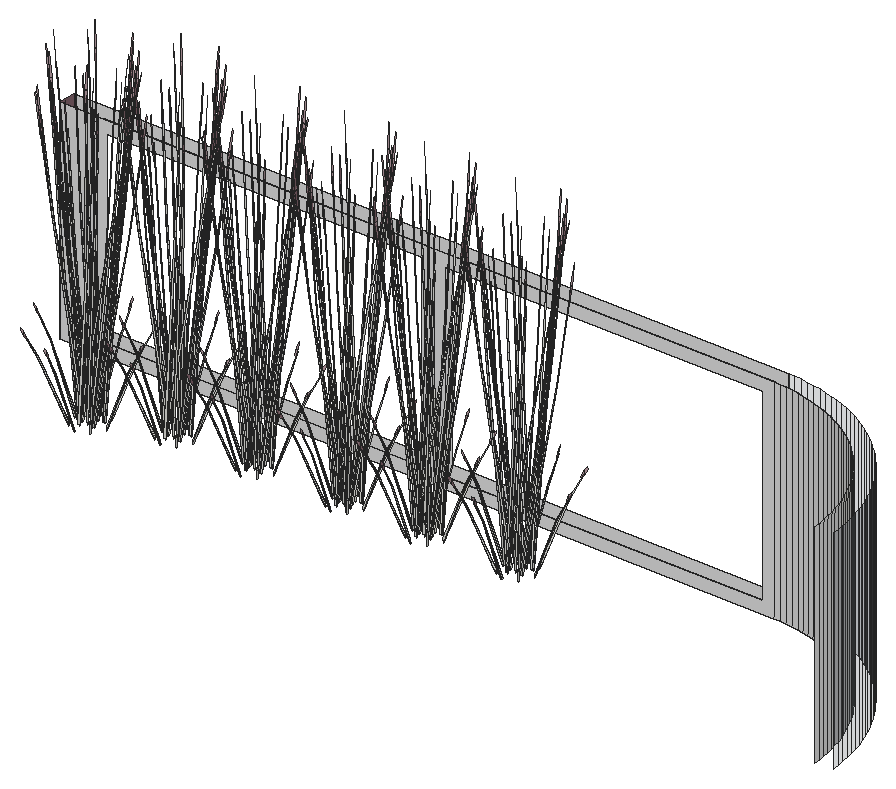
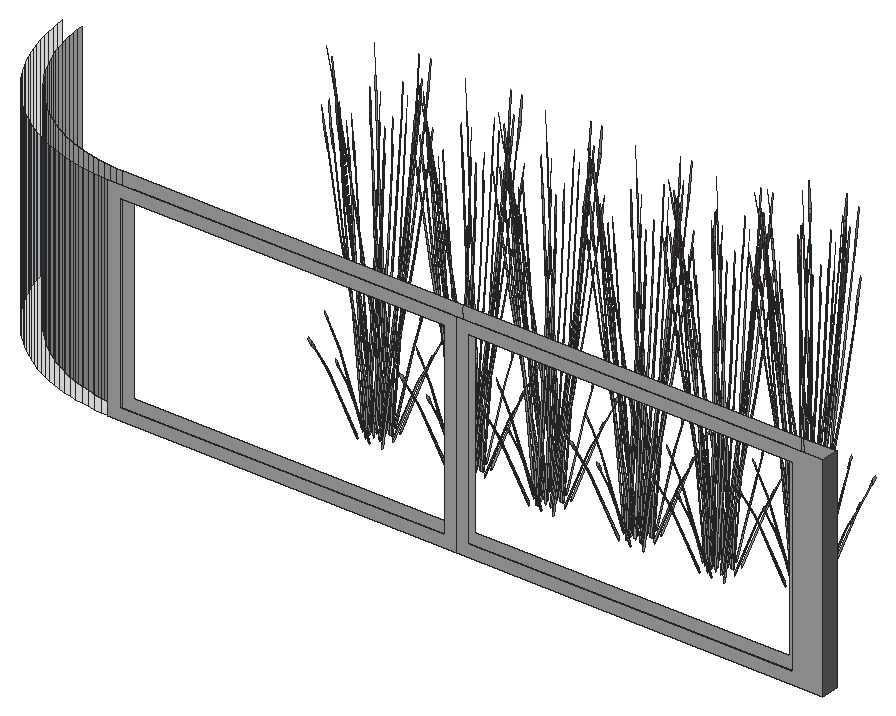
# SketchUp Ruby script. Lengths in inches.
U = 1.inch
M = Sketchup.active_model
def pt(a) = Geom::Point3d.new(a.map { |v| v * U })
def face(e, loops, mat)
  f = e.add_face(loops[0].map { |a| pt(a) })
  loops[1..].each { |l| e.add_face(l.map { |a| pt(a) }).erase! }
  f.material = f.back_material = mat if mat
  f
end
# faces: each face lists its corners as indices into pts; further lists are holes
def faces(e, pts, list, mat = nil) = list.each { |f| face(e, (f[0].is_a?(Array) ? f : [f]).map { |l| l.map { |i| pts[i] } }, mat) }
# xy, xz, yz: faces in a plane at the given z, y or x. An outline is a flat list of corners, or four numbers for a rectangle; further outlines are holes
def ring(l) = l.size == 4 ? [[l[0], l[1]], [l[2], l[1]], [l[2], l[3]], [l[0], l[3]]] : l.each_slice(2).to_a
def flat(e, list, mat, &to3) = list.each { |f| face(e, (f[0].is_a?(Array) ? f : [f]).map { |l| ring(l).map { |u, v| to3.(u, v) } }, mat) }
def xy(e, z, list, mat = nil) = flat(e, list, mat) { |x, y| [x, y, z] }
def xz(e, y, list, mat = nil) = flat(e, list, mat) { |x, z| [x, y, z] }
def yz(e, x, list, mat = nil) = flat(e, list, mat) { |y, z| [x, y, z] }
def lines(e, pts, list) = list.each { |a, b| e.add_line(pt(pts[a]), pt(pts[b])) }
# prism: a flat outline (further loops are holes) pulled along v
def prism(e, loops, v, mat = nil)
  f = face(e, loops, mat); d = Geom::Vector3d.new(v.map { |x| x * U })
  f.pushpull(f.normal.samedirection?(d) ? d.length : -d.length)
end
def box(e, o, s, mat = nil) = prism(e, [[o, [o[0] + s[0], o[1], o[2]], [o[0] + s[0], o[1] + s[1], o[2]], [o[0], o[1] + s[1], o[2]]]], [0, 0, s[2]], mat)
def at(x, y, z, deg = 0) = Geom::Transformation.translation(pt([x, y, z])) * Geom::Transformation.rotation(ORIGIN, Z_AXIS, deg.degrees)
def axes(o, x, y, z) = Geom::Transformation.new([*x, 0, *y, 0, *z, 0, *pt(o).to_a, 1])
def part(name) = M.definitions.add(name)
# library, detail: a bought-in or finely detailed component or shape, given as its bounding box
def library(name, o, s) = part(name).tap { |d| box(d.entities, o, s) }
def detail(e, o, s) = box(e.add_group.entities, o, s)
def put(e, d, t, mat = nil) = e.add_instance(d, t).tap { |i| i.material = mat if mat }
def group(e, t, mat = nil) = e.add_group.tap { |g| g.transformation = t; g.material = mat if mat }.entities
root = M.entities
M.materials.add("Glass_Basic_01").color = [105, 113, 122]
M.materials["Glass_Basic_01"].alpha = 0.25
M.materials.add("LightPink_Translucent").color = [144, 107, 117]
M.materials["LightPink_Translucent"].alpha = 0.75
M.materials.add("M01_Silver_Fog").color = [224, 224, 224]
M.materials.add("M06_Steel_Smoke").color = [114, 114, 114]
c1 = part("blade")
p = [[2.15,0.21,22],[0,0.17,0],[0.09,0.45,0],[2.18,0.31,22],[2.29,0.31,22],[0.38,0.45,0],
  [2.48,0.24,33],[2.49,0.24,33],[2.48,0.22,33]]
faces(c1.entities,p,[[0,1,2,3],[4,5,2,3],[6,3,4,7],[8,0,3,6]])
c2 = part("seeds")
p = [[0.3,-0.1,1.38],[-0.01,-0.03,1.59],[-0.01,-0.03,0.03],[0.14,-0.07,-0.07],[0.29,-0.03,3],[0.15,0.01,3.11]]
faces(c2.entities,p,[[0,1,2,3],[1,0,4,5]],"LightPink_Translucent")
c3 = part("blade with seeds")
put(c3.entities,c1,at(0,0,0))
put(c3.entities,c2,axes([2.4,0.25,30.99],[1.5799,-0.05474,1.17369],[-0.12525,1.92788,0.29478],[-0.07173,-0.02425,1.56792]))
xz(root,465.98,[[355.17,396,355.18,432]],"Glass_Basic_01")
xz(root,474,[[210,396,215.53,432],[215.53,396,216,432],[[216,396,273.49,432],[218,398,271.49,430]],[[273.49,396,331.45,432],[275.49,398,329.45,430]]],"M01_Silver_Fog")
xz(root,477,[[[210,396,272.25,432],[215,398,270.25,430]],[[272.25,396,331.5,432],[274.25,398,329.5,430]]],"M01_Silver_Fog")
yz(root,210,[[474,396,477,432]],"M06_Steel_Smoke")
yz(root,358.13,[[462.03,396,462.04,432]],"Glass_Basic_01")
p = [[360.01,447.89,396],[360.11,446.78,396],[360.11,446.78,432],[360.01,447.89,432],[363.1,447,396],[362.99,448.22,396],
  [362.99,448.22,432],[363.1,447,432],[359.87,449,396],[359.87,449,432],[362.83,449.44,396],[362.83,449.44,432],
  [359.68,450.1,396],[359.68,450.1,432],[362.63,450.66,396],[362.63,450.66,432],[359.45,451.2,396],[359.45,451.2,432],
  [362.38,451.86,396],[362.38,451.86,432],[359.18,452.28,396],[359.18,452.28,432],[362.08,453.06,396],[362.08,453.06,432],
  [358.875,453.35,396],[358.875,453.35,432],[361.74,454.24,396],[361.74,454.24,432],[358.52,454.41,396],[358.52,454.41,432],
  [361.35,455.41,396],[361.35,455.41,432],[358.13,455.46,396],[358.13,455.46,432],[360.92,456.5625,396],[360.92,456.5625,432],
  [357.7,456.49,396],[357.7,456.49,432],[357.23,457.5,396],[357.23,457.5,432],[360.45,457.7,396],[360.45,457.7,432],
  [356.73,458.5,396],[356.73,458.5,432],[359.93,458.82,396],[359.93,458.82,432],[356.18,459.47,396],[356.18,459.47,432],
  [359.37,459.91,396],[359.37,459.91,432],[355.6,460.43,396],[355.6,460.43,432],[358.77,460.99,396],[358.77,460.99,432],
  [354.98,461.36,396],[354.98,461.36,432],[358.13,462.03,396],[358.13,462.03,432],[354.33,462.26,396],[354.33,462.26,432],
  [358.13,462.04,396],[357.45,463.0625,396],[357.45,463.0625,432],[358.13,462.04,432],[353.64,463.14,396],[353.64,463.14,432],
  [352.92,464,396],[352.92,464,432],[356.73,464.0625,396],[356.73,464.0625,432],[352.17,464.83,396],[352.17,464.83,432],
  [355.97,465.03,396],[355.97,465.03,432],[351.39,465.62,396],[351.39,465.62,432],[355.18,465.98,396],[355.18,465.98,432],
  [350.58,466.39,396],[350.58,466.39,432],[355.17,465.98,396],[354.35,466.89,396],[354.35,466.89,432],[355.17,465.98,432],
  [349.74,467.125,396],[349.74,467.125,432],[353.49,467.76,396],[353.49,467.76,432],[348.87,467.83,396],[348.87,467.83,432],
  [347.97,468.5,396],[347.97,468.5,432],[352.59,468.61,396],[352.59,468.61,432],[347.05,469.13,396],[347.05,469.13,432],
  [351.67,469.42,396],[351.67,469.42,432],[346.11,469.73,396],[346.11,469.73,432],[350.71,470.19,396],[350.71,470.19,432],
  [345.15,470.29,396],[345.15,470.29,432],[349.72,470.93,396],[349.72,470.93,432],[344.16,470.82,396],[344.16,470.82,432],
  [343.16,471.3,396],[343.16,471.3,432],[348.71,471.63,396],[348.71,471.63,432],[342.13,471.75,396],[342.13,471.75,432],
  [347.67,472.29,396],[347.67,472.29,432],[341.09,472.16,396],[341.09,472.16,432],[340.04,472.53,396],[340.04,472.53,432],
  [346.61,472.91,396],[346.61,472.91,432],[338.97,472.86,396],[338.97,472.86,432],[337.89,473.15,396],[337.89,473.15,432],
  [345.52,473.49,396],[345.52,473.49,432],[336.8,473.4,396],[336.8,473.4,432],[335.71,473.6,396],[335.71,473.6,432],
  [344.41,474.03,396],[344.41,474.03,432],[334.6,473.77,396],[334.6,473.77,432],[333.49,473.89,396],[333.49,473.89,432],
  [332.38,473.97,396],[332.38,473.97,432],[331.45,474,396],[331.45,474,432],[343.29,474.52,396],[343.29,474.52,432],
  [342.14,474.97,396],[342.14,474.97,432],[340.98,475.38,396],[340.98,475.38,432],[339.8,475.75,396],[339.8,475.75,432],
  [338.61,476.0625,396],[338.61,476.0625,432],[337.41,476.34,396],[337.41,476.34,432],[336.2,476.5625,396],[336.2,476.5625,432],
  [334.99,476.74,396],[334.99,476.74,432],[333.76,476.88,396],[333.76,476.88,432],[332.53,476.97,396],[332.53,476.97,432],
  [331.5,477,396],[331.5,477,432]]
faces(root,p,[[0,1,2,3],[8,0,3,9],[12,8,9,13],[16,12,13,17],[20,16,17,21],[24,20,21,25],[28,24,25,29],[32,28,29,33],
  [36,32,33,37],[38,36,37,39],[42,38,39,43],[46,42,43,47],[50,46,47,51],[54,50,51,55],[58,54,55,59],[64,58,59,65],
  [66,64,65,67],[70,66,67,71],[74,70,71,75],[78,74,75,79],[84,78,79,85],[88,84,85,89],[90,88,89,91],[94,90,91,95],
  [98,94,95,99],[102,98,99,103],[106,102,103,107],[108,106,107,109],[112,108,109,113],[116,112,113,117],[118,116,117,119],[122,118,119,123],
  [124,122,123,125],[128,124,125,129],[130,128,129,131],[134,130,131,135],[136,134,135,137],[138,136,137,139],[140,138,139,141]],"M01_Silver_Fog")
faces(root,p,[[4,5,6,7],[5,10,11,6],[10,14,15,11],[14,18,19,15],[18,22,23,19],[22,26,27,23],[26,30,31,27],[30,34,35,31],
  [34,40,41,35],[40,44,45,41],[44,48,49,45],[48,52,53,49],[52,56,57,53],[60,61,62,63],[61,68,69,62],[68,72,73,69],
  [72,76,77,73],[80,81,82,83],[81,86,87,82],[86,92,93,87],[92,96,97,93],[96,100,101,97],[100,104,105,101],[104,110,111,105],
  [110,114,115,111],[114,120,121,115],[120,126,127,121],[126,132,133,127],[132,142,143,133],[142,144,145,143],[144,146,147,145],[146,148,149,147],
  [148,150,151,149],[150,152,153,151],[152,154,155,153],[154,156,157,155],[156,158,159,157],[158,160,161,159],[160,162,163,161]],"Glass_Basic_01")
put(root,c3,axes([228.93,453.59,397.49],[-0.08428,0.0194,1.76342],[-0.46606,-0.21841,-0.26939],[0.00782,-0.18218,0.30037]))
put(root,c3,axes([227.42,454.26,397.49],[-0.04867,0.07094,1.76342],[-0.49185,0.15296,-0.26939],[-0.11882,-0.13915,0.30037]))
put(root,c3,axes([228.23,456.2,398.1],[-0.20635,-0.55225,-0.69835],[0.59439,-0.19889,-0.18329],[-0.02281,-0.18701,1.54149]))
put(root,c3,axes([230.99,454.52,397.49],[-0.0752,-0.04243,1.76342],[-0.19317,-0.47398,-0.26939],[0.13031,-0.12863,0.30037]))
put(root,c3,axes([227.01,456.13,398.02],[0,-0.53854,-0.49651],[0.56215,0,0],[0,-0.12266,1.57504]))
put(root,c3,axes([228.58,454.53,398.02],[0.47024,-0.26927,-0.49651],[0.28107,0.48284,0],[0.1071,-0.06133,1.57504]))
put(root,c3,axes([229.13,455.64,398.06],[0.33843,-0.40479,-0.62353],[0.42041,0.36705,-0.16365],[0.13561,-0.10098,1.37633]))
put(root,c3,axes([228.54,456.35,398.21],[0.24378,-0.48527,-0.44739],[0.50654,0.23354,0.21531],[0,-0.11186,1.43643]))
put(root,c3,axes([228.77,456.11,398.67],[-0.05855,-0.61451,-0.29095],[0.60981,-0.03716,-0.50002],[0.10738,-0.08185,1.59708]))
put(root,c3,axes([227.26,456.14,398.03],[0.35073,-0.33601,-0.30978],[0.35073,0.33601,0.30978],[0,-0.10823,1.38974]))
put(root,c3,axes([228.48,456.75,398.67],[-0.56585,-0.25696,-0.29095],[0.27246,-0.54236,-0.50002],[-0.01778,-0.13316,1.59708]))
put(root,c3,axes([228.6875,454.75,398.03],[0.46876,0.13325,-0.30978],[-0.11803,0.46926,0.30978],[0.0945,-0.05411,1.38974]))
put(root,c3,axes([240.17,457.83,397.49],[-0.08428,0.0194,1.76342],[-0.46606,-0.21841,-0.26939],[0.00782,-0.18218,0.30037]))
put(root,c3,axes([253.88,457.83,397.49],[-0.08428,0.0194,1.76342],[-0.46606,-0.21841,-0.26939],[0.00782,-0.18218,0.30037]))
put(root,c3,axes([269.125,457.83,397.49],[-0.08428,0.0194,1.76342],[-0.46606,-0.21841,-0.26939],[0.00782,-0.18218,0.30037]))
put(root,c3,axes([282.74,457.83,397.49],[-0.08428,0.0194,1.76342],[-0.46606,-0.21841,-0.26939],[0.00782,-0.18218,0.30037]))
put(root,c3,axes([298.27,457.83,397.49],[-0.08428,0.0194,1.76342],[-0.46606,-0.21841,-0.26939],[0.00782,-0.18218,0.30037]))
put(root,c3,axes([228.58,457.0625,398.21],[-0.30184,-0.45202,-0.44739],[0.45719,-0.31831,0.21531],[-0.09768,-0.05593,1.43643]))
put(root,c3,axes([228.3125,457.24,398.06],[-0.52267,-0.08829,-0.62353],[0.11029,-0.54463,-0.16365],[-0.15598,-0.06599,1.37633]))
put(root,c3,axes([228.19,455.71,397.59],[-0.49456,0.21561,1.28929],[-0.15741,-0.61865,0.50096],[0.30369,0.01029,1.46642]))
put(root,c3,axes([238.66,458.5,397.49],[-0.04867,0.07094,1.76342],[-0.49185,0.15296,-0.26939],[-0.11882,-0.13915,0.30037]))
put(root,c3,axes([252.37,458.5,397.49],[-0.04867,0.07094,1.76342],[-0.49185,0.15296,-0.26939],[-0.11882,-0.13915,0.30037]))
put(root,c3,axes([267.62,458.5,397.49],[-0.04867,0.07094,1.76342],[-0.49185,0.15296,-0.26939],[-0.11882,-0.13915,0.30037]))
put(root,c3,axes([281.23,458.5,397.49],[-0.04867,0.07094,1.76342],[-0.49185,0.15296,-0.26939],[-0.11882,-0.13915,0.30037]))
put(root,c3,axes([296.76,458.5,397.49],[-0.04867,0.07094,1.76342],[-0.49185,0.15296,-0.26939],[-0.11882,-0.13915,0.30037]))
put(root,c3,axes([232.05,456.55,397.49],[-0.02626,-0.08176,1.76342],[0.18213,-0.47826,-0.26939],[0.18372,-0.00688,0.30037]))
put(root,c3,axes([239.48,460.45,398.1],[-0.20635,-0.55225,-0.69835],[0.59439,-0.19889,-0.18329],[-0.02281,-0.18701,1.54149]))
put(root,c3,axes([253.18,460.45,398.1],[-0.20635,-0.55225,-0.69835],[0.59439,-0.19889,-0.18329],[-0.02281,-0.18701,1.54149]))
put(root,c3,axes([268.43,460.45,398.1],[-0.20635,-0.55225,-0.69835],[0.59439,-0.19889,-0.18329],[-0.02281,-0.18701,1.54149]))
put(root,c3,axes([282.04,460.45,398.1],[-0.20635,-0.55225,-0.69835],[0.59439,-0.19889,-0.18329],[-0.02281,-0.18701,1.54149]))
put(root,c3,axes([297.58,460.45,398.1],[-0.20635,-0.55225,-0.69835],[0.59439,-0.19889,-0.18329],[-0.02281,-0.18701,1.54149]))
put(root,c3,axes([242.23,458.76,397.49],[-0.0752,-0.04243,1.76342],[-0.19317,-0.47398,-0.26939],[0.13031,-0.12863,0.30037]))
put(root,c3,axes([255.94,458.76,397.49],[-0.0752,-0.04243,1.76342],[-0.19317,-0.47398,-0.26939],[0.13031,-0.12863,0.30037]))
put(root,c3,axes([271.19,458.76,397.49],[-0.0752,-0.04243,1.76342],[-0.19317,-0.47398,-0.26939],[0.13031,-0.12863,0.30037]))
put(root,c3,axes([284.8,458.76,397.49],[-0.0752,-0.04243,1.76342],[-0.19317,-0.47398,-0.26939],[0.13031,-0.12863,0.30037]))
put(root,c3,axes([300.33,458.76,397.49],[-0.0752,-0.04243,1.76342],[-0.19317,-0.47398,-0.26939],[0.13031,-0.12863,0.30037]))
put(root,c3,axes([226.63,456.47,397.49],[0.01274,0.08487,1.76342],[-0.25688,0.44323,-0.26939],[-0.18246,-0.02234,0.30037]))
put(root,c3,axes([227.76,458.07,398.03],[-0.11803,-0.46926,-0.30978],[0.46876,-0.13325,0.30978],[-0.0945,-0.05411,1.38974]))
put(root,c3,axes([229.47,456.03,398.67],[0.5073,-0.35754,-0.29095],[0.33735,0.5052,-0.50002],[0.12516,0.05131,1.59708]))
put(root,c3,axes([227.625,458.27,398.02],[-0.47024,-0.26927,-0.49651],[0.28107,-0.48284,0],[-0.1071,-0.06133,1.57504]))
put(root,c3,axes([230.75,455.08,398.02],[0.47024,0.26927,-0.49651],[-0.28107,0.48284,0],[0.1071,0.06133,1.57504]))
put(root,c3,axes([228.9,457.32,398.67],[-0.5073,0.35754,-0.29095],[-0.33735,-0.5052,-0.50002],[-0.12516,-0.05131,1.59708]))
put(root,c3,axes([230.62,455.28,398.03],[0.11803,0.46926,-0.30978],[-0.46876,0.13325,0.30978],[0.0945,0.05411,1.38974]))
put(root,c3,axes([238.26,460.375,398.02],[0,-0.53854,-0.49651],[0.56215,0,0],[0,-0.12266,1.57504]))
put(root,c3,axes([251.97,460.375,398.02],[0,-0.53854,-0.49651],[0.56215,0,0],[0,-0.12266,1.57504]))
put(root,c3,axes([267.22,460.375,398.02],[0,-0.53854,-0.49651],[0.56215,0,0],[0,-0.12266,1.57504]))
put(root,c3,axes([280.83,460.375,398.02],[0,-0.53854,-0.49651],[0.56215,0,0],[0,-0.12266,1.57504]))
put(root,c3,axes([296.36,460.375,398.02],[0,-0.53854,-0.49651],[0.56215,0,0],[0,-0.12266,1.57504]))
put(root,c3,axes([239.82,458.78,398.02],[0.47024,-0.26927,-0.49651],[0.28107,0.48284,0],[0.1071,-0.06133,1.57504]))
put(root,c3,axes([253.53,458.78,398.02],[0.47024,-0.26927,-0.49651],[0.28107,0.48284,0],[0.1071,-0.06133,1.57504]))
put(root,c3,axes([268.78,458.78,398.02],[0.47024,-0.26927,-0.49651],[0.28107,0.48284,0],[0.1071,-0.06133,1.57504]))
put(root,c3,axes([282.39,458.78,398.02],[0.47024,-0.26927,-0.49651],[0.28107,0.48284,0],[0.1071,-0.06133,1.57504]))
put(root,c3,axes([297.92,458.78,398.02],[0.47024,-0.26927,-0.49651],[0.28107,0.48284,0],[0.1071,-0.06133,1.57504]))
put(root,c3,axes([230.0625,456.11,398.06],[0.52267,0.08829,-0.62353],[-0.11029,0.54463,-0.16365],[0.15598,0.06599,1.37633]))
put(root,c3,axes([240.38,459.88,398.06],[0.33843,-0.40479,-0.62353],[0.42041,0.36705,-0.16365],[0.13561,-0.10098,1.37633]))
put(root,c3,axes([254.09,459.88,398.06],[0.33843,-0.40479,-0.62353],[0.42041,0.36705,-0.16365],[0.13561,-0.10098,1.37633]))
put(root,c3,axes([269.33,459.88,398.06],[0.33843,-0.40479,-0.62353],[0.42041,0.36705,-0.16365],[0.13561,-0.10098,1.37633]))
put(root,c3,axes([282.95,459.88,398.06],[0.33843,-0.40479,-0.62353],[0.42041,0.36705,-0.16365],[0.13561,-0.10098,1.37633]))
put(root,c3,axes([298.48,459.88,398.06],[0.33843,-0.40479,-0.62353],[0.42041,0.36705,-0.16365],[0.13561,-0.10098,1.37633]))
put(root,c3,axes([239.79,460.59,398.21],[0.24378,-0.48527,-0.44739],[0.50654,0.23354,0.21531],[0,-0.11186,1.43643]))
put(root,c3,axes([253.5,460.59,398.21],[0.24378,-0.48527,-0.44739],[0.50654,0.23354,0.21531],[0,-0.11186,1.43643]))
put(root,c3,axes([268.75,460.59,398.21],[0.24378,-0.48527,-0.44739],[0.50654,0.23354,0.21531],[0,-0.11186,1.43643]))
put(root,c3,axes([282.36,460.59,398.21],[0.24378,-0.48527,-0.44739],[0.50654,0.23354,0.21531],[0,-0.11186,1.43643]))
put(root,c3,axes([297.89,460.59,398.21],[0.24378,-0.48527,-0.44739],[0.50654,0.23354,0.21531],[0,-0.11186,1.43643]))
put(root,c3,axes([238.5,460.39,398.03],[0.35073,-0.33601,-0.30978],[0.35073,0.33601,0.30978],[0,-0.10823,1.38974]))
put(root,c3,axes([252.21,460.39,398.03],[0.35073,-0.33601,-0.30978],[0.35073,0.33601,0.30978],[0,-0.10823,1.38974]))
put(root,c3,axes([267.46,460.39,398.03],[0.35073,-0.33601,-0.30978],[0.35073,0.33601,0.30978],[0,-0.10823,1.38974]))
put(root,c3,axes([281.07,460.39,398.03],[0.35073,-0.33601,-0.30978],[0.35073,0.33601,0.30978],[0,-0.10823,1.38974]))
put(root,c3,axes([296.6,460.39,398.03],[0.35073,-0.33601,-0.30978],[0.35073,0.33601,0.30978],[0,-0.10823,1.38974]))
put(root,c3,axes([229.79,456.28,398.21],[0.30184,0.45202,-0.44739],[-0.45719,0.31831,0.21531],[0.09768,0.05593,1.43643]))
put(root,c3,axes([239.93,458.99,398.03],[0.46876,0.13325,-0.30978],[-0.11803,0.46926,0.30978],[0.0945,-0.05411,1.38974]))
put(root,c3,axes([253.64,458.99,398.03],[0.46876,0.13325,-0.30978],[-0.11803,0.46926,0.30978],[0.0945,-0.05411,1.38974]))
put(root,c3,axes([268.89,458.99,398.03],[0.46876,0.13325,-0.30978],[-0.11803,0.46926,0.30978],[0.0945,-0.05411,1.38974]))
put(root,c3,axes([282.5,458.99,398.03],[0.46876,0.13325,-0.30978],[-0.11803,0.46926,0.30978],[0.0945,-0.05411,1.38974]))
put(root,c3,axes([298.03,458.99,398.03],[0.46876,0.13325,-0.30978],[-0.11803,0.46926,0.30978],[0.0945,-0.05411,1.38974]))
put(root,c3,axes([229.23,457.39,398.21],[-0.54562,0.03324,-0.44739],[-0.04934,-0.55185,0.21531],[-0.09768,0.05593,1.43643]))
put(root,c3,axes([229.6875,458.6,398.03],[-0.46876,-0.13325,-0.30978],[0.11803,-0.46926,0.30978],[-0.0945,0.05411,1.38974]))
put(root,c3,axes([229.89,456.59,398.67],[0.56585,0.25696,-0.29095],[-0.27246,0.54236,-0.50002],[0.01778,0.13316,1.59708]))
put(root,c3,axes([239.83,461.31,398.21],[-0.30184,-0.45202,-0.44739],[0.45719,-0.31831,0.21531],[-0.09768,-0.05593,1.43643]))
put(root,c3,axes([253.53,461.31,398.21],[-0.30184,-0.45202,-0.44739],[0.45719,-0.31831,0.21531],[-0.09768,-0.05593,1.43643]))
put(root,c3,axes([268.78,461.31,398.21],[-0.30184,-0.45202,-0.44739],[0.45719,-0.31831,0.21531],[-0.09768,-0.05593,1.43643]))
put(root,c3,axes([282.4,461.31,398.21],[-0.30184,-0.45202,-0.44739],[0.45719,-0.31831,0.21531],[-0.09768,-0.05593,1.43643]))
put(root,c3,axes([297.93,461.31,398.21],[-0.30184,-0.45202,-0.44739],[0.45719,-0.31831,0.21531],[-0.09768,-0.05593,1.43643]))
put(root,c3,axes([231.12,457.2,398.03],[-0.35073,0.33601,-0.30978],[-0.35073,-0.33601,0.30978],[0,0.10823,1.38974]))
put(root,c3,axes([229.61,457.24,398.67],[0.05855,0.61451,-0.29095],[-0.60981,0.03716,-0.50002],[-0.10738,0.08185,1.59708]))
put(root,c3,axes([229.83,457,398.21],[-0.24378,0.48527,-0.44739],[-0.50654,-0.23354,0.21531],[0,0.11186,1.43643]))
put(root,c3,axes([229.24,457.71,398.06],[-0.33843,0.40479,-0.62353],[-0.42041,-0.36705,-0.16365],[-0.13561,0.10098,1.37633]))
put(root,c3,axes([239.56,461.48,398.06],[-0.52267,-0.08829,-0.62353],[0.11029,-0.54463,-0.16365],[-0.15598,-0.06599,1.37633]))
put(root,c3,axes([253.26,461.48,398.06],[-0.52267,-0.08829,-0.62353],[0.11029,-0.54463,-0.16365],[-0.15598,-0.06599,1.37633]))
put(root,c3,axes([268.51,461.48,398.06],[-0.52267,-0.08829,-0.62353],[0.11029,-0.54463,-0.16365],[-0.15598,-0.06599,1.37633]))
put(root,c3,axes([282.125,461.48,398.06],[-0.52267,-0.08829,-0.62353],[0.11029,-0.54463,-0.16365],[-0.15598,-0.06599,1.37633]))
put(root,c3,axes([297.66,461.48,398.06],[-0.52267,-0.08829,-0.62353],[0.11029,-0.54463,-0.16365],[-0.15598,-0.06599,1.37633]))
put(root,c3,axes([229.8,458.8125,398.02],[-0.47024,0.26927,-0.49651],[-0.28107,-0.48284,0],[-0.1071,0.06133,1.57504]))
put(root,c3,axes([231.36,457.22,398.02],[0,0.53854,-0.49651],[-0.56215,0,0],[0,0.12266,1.57504]))
put(root,c3,axes([239.44,459.96,397.59],[-0.49456,0.21561,1.28929],[-0.15741,-0.61865,0.50096],[0.30369,0.01029,1.46642]))
put(root,c3,axes([253.14,459.96,397.59],[-0.49456,0.21561,1.28929],[-0.15741,-0.61865,0.50096],[0.30369,0.01029,1.46642]))
put(root,c3,axes([268.39,459.96,397.59],[-0.49456,0.21561,1.28929],[-0.15741,-0.61865,0.50096],[0.30369,0.01029,1.46642]))
put(root,c3,axes([282,459.96,397.59],[-0.49456,0.21561,1.28929],[-0.15741,-0.61865,0.50096],[0.30369,0.01029,1.46642]))
put(root,c3,axes([297.53,459.96,397.59],[-0.49456,0.21561,1.28929],[-0.15741,-0.61865,0.50096],[0.30369,0.01029,1.46642]))
put(root,c3,axes([243.3,460.8,397.49],[-0.02626,-0.08176,1.76342],[0.18213,-0.47826,-0.26939],[0.18372,-0.00688,0.30037]))
put(root,c3,axes([257.01,460.8,397.49],[-0.02626,-0.08176,1.76342],[0.18213,-0.47826,-0.26939],[0.18372,-0.00688,0.30037]))
put(root,c3,axes([272.25,460.8,397.49],[-0.02626,-0.08176,1.76342],[0.18213,-0.47826,-0.26939],[0.18372,-0.00688,0.30037]))
put(root,c3,axes([285.87,460.8,397.49],[-0.02626,-0.08176,1.76342],[0.18213,-0.47826,-0.26939],[0.18372,-0.00688,0.30037]))
put(root,c3,axes([301.4,460.8,397.49],[-0.02626,-0.08176,1.76342],[0.18213,-0.47826,-0.26939],[0.18372,-0.00688,0.30037]))
put(root,c3,axes([237.875,460.71,397.49],[0.01274,0.08487,1.76342],[-0.25688,0.44323,-0.26939],[-0.18246,-0.02234,0.30037]))
put(root,c3,axes([251.58,460.71,397.49],[0.01274,0.08487,1.76342],[-0.25688,0.44323,-0.26939],[-0.18246,-0.02234,0.30037]))
put(root,c3,axes([266.83,460.71,397.49],[0.01274,0.08487,1.76342],[-0.25688,0.44323,-0.26939],[-0.18246,-0.02234,0.30037]))
put(root,c3,axes([280.45,460.71,397.49],[0.01274,0.08487,1.76342],[-0.25688,0.44323,-0.26939],[-0.18246,-0.02234,0.30037]))
put(root,c3,axes([295.98,460.71,397.49],[0.01274,0.08487,1.76342],[-0.25688,0.44323,-0.26939],[-0.18246,-0.02234,0.30037]))
put(root,c3,axes([239,462.3125,398.03],[-0.11803,-0.46926,-0.30978],[0.46876,-0.13325,0.30978],[-0.0945,-0.05411,1.38974]))
put(root,c3,axes([252.71,462.3125,398.03],[-0.11803,-0.46926,-0.30978],[0.46876,-0.13325,0.30978],[-0.0945,-0.05411,1.38974]))
put(root,c3,axes([267.96,462.3125,398.03],[-0.11803,-0.46926,-0.30978],[0.46876,-0.13325,0.30978],[-0.0945,-0.05411,1.38974]))
put(root,c3,axes([281.57,462.3125,398.03],[-0.11803,-0.46926,-0.30978],[0.46876,-0.13325,0.30978],[-0.0945,-0.05411,1.38974]))
put(root,c3,axes([297.1,462.3125,398.03],[-0.11803,-0.46926,-0.30978],[0.46876,-0.13325,0.30978],[-0.0945,-0.05411,1.38974]))
put(root,c3,axes([230.73,458.91,397.49],[0.03661,-0.07775,1.76342],[0.46087,-0.22898,-0.26939],[0.13972,0.11851,0.30037]))
put(root,c3,axes([238.87,462.51,398.02],[-0.47024,-0.26927,-0.49651],[0.28107,-0.48284,0],[-0.1071,-0.06133,1.57504]))
put(root,c3,axes([252.58,462.51,398.02],[-0.47024,-0.26927,-0.49651],[0.28107,-0.48284,0],[-0.1071,-0.06133,1.57504]))
put(root,c3,axes([267.83,462.51,398.02],[-0.47024,-0.26927,-0.49651],[0.28107,-0.48284,0],[-0.1071,-0.06133,1.57504]))
put(root,c3,axes([281.44,462.51,398.02],[-0.47024,-0.26927,-0.49651],[0.28107,-0.48284,0],[-0.1071,-0.06133,1.57504]))
put(root,c3,axes([296.97,462.51,398.02],[-0.47024,-0.26927,-0.49651],[0.28107,-0.48284,0],[-0.1071,-0.06133,1.57504]))
put(root,c3,axes([230.12,457.14,398.09],[0.18424,0.49308,-0.69212],[-0.53071,0.17758,-0.18165],[0.02036,0.16697,1.52773]))
put(root,c3,axes([241.99,459.32,398.02],[0.47024,0.26927,-0.49651],[-0.28107,0.48284,0],[0.1071,0.06133,1.57504]))
put(root,c3,axes([255.7,459.32,398.02],[0.47024,0.26927,-0.49651],[-0.28107,0.48284,0],[0.1071,0.06133,1.57504]))
put(root,c3,axes([270.95,459.32,398.02],[0.47024,0.26927,-0.49651],[-0.28107,0.48284,0],[0.1071,0.06133,1.57504]))
put(root,c3,axes([284.5625,459.32,398.02],[0.47024,0.26927,-0.49651],[-0.28107,0.48284,0],[0.1071,0.06133,1.57504]))
put(root,c3,axes([300.09,459.32,398.02],[0.47024,0.26927,-0.49651],[-0.28107,0.48284,0],[0.1071,0.06133,1.57504]))
put(root,c3,axes([226.49,458.84,397.49],[0.0674,0.0538,1.76342],[0.11428,0.49852,-0.26939],[-0.14937,0.10631,0.30037]))
put(root,c3,axes([241.86,459.53,398.03],[0.11803,0.46926,-0.30978],[-0.46876,0.13325,0.30978],[0.0945,0.05411,1.38974]))
put(root,c3,axes([255.57,459.53,398.03],[0.11803,0.46926,-0.30978],[-0.46876,0.13325,0.30978],[0.0945,0.05411,1.38974]))
put(root,c3,axes([270.82,459.53,398.03],[0.11803,0.46926,-0.30978],[-0.46876,0.13325,0.30978],[0.0945,0.05411,1.38974]))
put(root,c3,axes([284.43,459.53,398.03],[0.11803,0.46926,-0.30978],[-0.46876,0.13325,0.30978],[0.0945,0.05411,1.38974]))
put(root,c3,axes([299.96,459.53,398.03],[0.11803,0.46926,-0.30978],[-0.46876,0.13325,0.30978],[0.0945,0.05411,1.38974]))
put(root,c3,axes([241.31,460.36,398.06],[0.52267,0.08829,-0.62353],[-0.11029,0.54463,-0.16365],[0.15598,0.06599,1.37633]))
put(root,c3,axes([255.02,460.36,398.06],[0.52267,0.08829,-0.62353],[-0.11029,0.54463,-0.16365],[0.15598,0.06599,1.37633]))
put(root,c3,axes([270.26,460.36,398.06],[0.52267,0.08829,-0.62353],[-0.11029,0.54463,-0.16365],[0.15598,0.06599,1.37633]))
put(root,c3,axes([283.88,460.36,398.06],[0.52267,0.08829,-0.62353],[-0.11029,0.54463,-0.16365],[0.15598,0.06599,1.37633]))
put(root,c3,axes([299.41,460.36,398.06],[0.52267,0.08829,-0.62353],[-0.11029,0.54463,-0.16365],[0.15598,0.06599,1.37633]))
put(root,c3,axes([228.57,458.89,397.49],[0.08132,-0.0293,1.76342],[0.48914,0.1613,-0.26939],[0.0143,0.18179,0.30037]))
put(root,c3,axes([241.04,460.53,398.21],[0.30184,0.45202,-0.44739],[-0.45719,0.31831,0.21531],[0.09768,0.05593,1.43643]))
put(root,c3,axes([254.75,460.53,398.21],[0.30184,0.45202,-0.44739],[-0.45719,0.31831,0.21531],[0.09768,0.05593,1.43643]))
put(root,c3,axes([269.99,460.53,398.21],[0.30184,0.45202,-0.44739],[-0.45719,0.31831,0.21531],[0.09768,0.05593,1.43643]))
put(root,c3,axes([283.61,460.53,398.21],[0.30184,0.45202,-0.44739],[-0.45719,0.31831,0.21531],[0.09768,0.05593,1.43643]))
put(root,c3,axes([299.14,460.53,398.21],[0.30184,0.45202,-0.44739],[-0.45719,0.31831,0.21531],[0.09768,0.05593,1.43643]))
put(root,c3,axes([240.47,461.63,398.21],[-0.54562,0.03324,-0.44739],[-0.04934,-0.55185,0.21531],[-0.09768,0.05593,1.43643]))
put(root,c3,axes([254.18,461.63,398.21],[-0.54562,0.03324,-0.44739],[-0.04934,-0.55185,0.21531],[-0.09768,0.05593,1.43643]))
put(root,c3,axes([269.43,461.63,398.21],[-0.54562,0.03324,-0.44739],[-0.04934,-0.55185,0.21531],[-0.09768,0.05593,1.43643]))
put(root,c3,axes([283.04,461.63,398.21],[-0.54562,0.03324,-0.44739],[-0.04934,-0.55185,0.21531],[-0.09768,0.05593,1.43643]))
put(root,c3,axes([298.57,461.63,398.21],[-0.54562,0.03324,-0.44739],[-0.04934,-0.55185,0.21531],[-0.09768,0.05593,1.43643]))
put(root,c3,axes([240.93,462.84,398.03],[-0.46876,-0.13325,-0.30978],[0.11803,-0.46926,0.30978],[-0.0945,0.05411,1.38974]))
put(root,c3,axes([254.64,462.84,398.03],[-0.46876,-0.13325,-0.30978],[0.11803,-0.46926,0.30978],[-0.0945,0.05411,1.38974]))
put(root,c3,axes([269.89,462.84,398.03],[-0.46876,-0.13325,-0.30978],[0.11803,-0.46926,0.30978],[-0.0945,0.05411,1.38974]))
put(root,c3,axes([283.5,462.84,398.03],[-0.46876,-0.13325,-0.30978],[0.11803,-0.46926,0.30978],[-0.0945,0.05411,1.38974]))
put(root,c3,axes([299.03,462.84,398.03],[-0.46876,-0.13325,-0.30978],[0.11803,-0.46926,0.30978],[-0.0945,0.05411,1.38974]))
put(root,c3,axes([241.14,460.84,398.67],[0.56585,0.25696,-0.29095],[-0.27246,0.54236,-0.50002],[0.01778,0.13316,1.59708]))
put(root,c3,axes([242.36,461.45,398.03],[-0.35073,0.33601,-0.30978],[-0.35073,-0.33601,0.30978],[0,0.10823,1.38974]))
put(root,c3,axes([256.07,461.45,398.03],[-0.35073,0.33601,-0.30978],[-0.35073,-0.33601,0.30978],[0,0.10823,1.38974]))
put(root,c3,axes([271.32,461.45,398.03],[-0.35073,0.33601,-0.30978],[-0.35073,-0.33601,0.30978],[0,0.10823,1.38974]))
put(root,c3,axes([284.93,461.45,398.03],[-0.35073,0.33601,-0.30978],[-0.35073,-0.33601,0.30978],[0,0.10823,1.38974]))
put(root,c3,axes([300.46,461.45,398.03],[-0.35073,0.33601,-0.30978],[-0.35073,-0.33601,0.30978],[0,0.10823,1.38974]))
put(root,c3,axes([240.85,461.48,398.67],[0.05855,0.61451,-0.29095],[-0.60981,0.03716,-0.50002],[-0.10738,0.08185,1.59708]))
put(root,c3,axes([241.08,461.24,398.21],[-0.24378,0.48527,-0.44739],[-0.50654,-0.23354,0.21531],[0,0.11186,1.43643]))
put(root,c3,axes([254.78,461.24,398.21],[-0.24378,0.48527,-0.44739],[-0.50654,-0.23354,0.21531],[0,0.11186,1.43643]))
put(root,c3,axes([270.03,461.24,398.21],[-0.24378,0.48527,-0.44739],[-0.50654,-0.23354,0.21531],[0,0.11186,1.43643]))
put(root,c3,axes([283.64,461.24,398.21],[-0.24378,0.48527,-0.44739],[-0.50654,-0.23354,0.21531],[0,0.11186,1.43643]))
put(root,c3,axes([299.17,461.24,398.21],[-0.24378,0.48527,-0.44739],[-0.50654,-0.23354,0.21531],[0,0.11186,1.43643]))
put(root,c3,axes([240.49,461.95,398.06],[-0.33843,0.40479,-0.62353],[-0.42041,-0.36705,-0.16365],[-0.13561,0.10098,1.37633]))
put(root,c3,axes([254.19,461.95,398.06],[-0.33843,0.40479,-0.62353],[-0.42041,-0.36705,-0.16365],[-0.13561,0.10098,1.37633]))
put(root,c3,axes([269.44,461.95,398.06],[-0.33843,0.40479,-0.62353],[-0.42041,-0.36705,-0.16365],[-0.13561,0.10098,1.37633]))
put(root,c3,axes([283.06,461.95,398.06],[-0.33843,0.40479,-0.62353],[-0.42041,-0.36705,-0.16365],[-0.13561,0.10098,1.37633]))
put(root,c3,axes([298.59,461.95,398.06],[-0.33843,0.40479,-0.62353],[-0.42041,-0.36705,-0.16365],[-0.13561,0.10098,1.37633]))
put(root,c3,axes([241.04,463.06,398.02],[-0.47024,0.26927,-0.49651],[-0.28107,-0.48284,0],[-0.1071,0.06133,1.57504]))
put(root,c3,axes([254.75,463.06,398.02],[-0.47024,0.26927,-0.49651],[-0.28107,-0.48284,0],[-0.1071,0.06133,1.57504]))
put(root,c3,axes([270,463.06,398.02],[-0.47024,0.26927,-0.49651],[-0.28107,-0.48284,0],[-0.1071,0.06133,1.57504]))
put(root,c3,axes([283.61,463.06,398.02],[-0.47024,0.26927,-0.49651],[-0.28107,-0.48284,0],[-0.1071,0.06133,1.57504]))
put(root,c3,axes([299.14,463.06,398.02],[-0.47024,0.26927,-0.49651],[-0.28107,-0.48284,0],[-0.1071,0.06133,1.57504]))
put(root,c3,axes([242.61,461.46,398.02],[0,0.53854,-0.49651],[-0.56215,0,0],[0,0.12266,1.57504]))
put(root,c3,axes([256.3125,461.46,398.02],[0,0.53854,-0.49651],[-0.56215,0,0],[0,0.12266,1.57504]))
put(root,c3,axes([271.5625,461.46,398.02],[0,0.53854,-0.49651],[-0.56215,0,0],[0,0.12266,1.57504]))
put(root,c3,axes([285.17,461.46,398.02],[0,0.53854,-0.49651],[-0.56215,0,0],[0,0.12266,1.57504]))
put(root,c3,axes([300.7,461.46,398.02],[0,0.53854,-0.49651],[-0.56215,0,0],[0,0.12266,1.57504]))
put(root,c3,axes([241.97,463.16,397.49],[0.03661,-0.07775,1.76342],[0.46087,-0.22898,-0.26939],[0.13972,0.11851,0.30037]))
put(root,c3,axes([255.68,463.16,397.49],[0.03661,-0.07775,1.76342],[0.46087,-0.22898,-0.26939],[0.13972,0.11851,0.30037]))
put(root,c3,axes([270.93,463.16,397.49],[0.03661,-0.07775,1.76342],[0.46087,-0.22898,-0.26939],[0.13972,0.11851,0.30037]))
put(root,c3,axes([284.54,463.16,397.49],[0.03661,-0.07775,1.76342],[0.46087,-0.22898,-0.26939],[0.13972,0.11851,0.30037]))
put(root,c3,axes([300.07,463.16,397.49],[0.03661,-0.07775,1.76342],[0.46087,-0.22898,-0.26939],[0.13972,0.11851,0.30037]))
put(root,c3,axes([241.36,461.39,398.09],[0.18424,0.49308,-0.69212],[-0.53071,0.17758,-0.18165],[0.02036,0.16697,1.52773]))
put(root,c3,axes([255.07,461.39,398.09],[0.18424,0.49308,-0.69212],[-0.53071,0.17758,-0.18165],[0.02036,0.16697,1.52773]))
put(root,c3,axes([270.32,461.39,398.09],[0.18424,0.49308,-0.69212],[-0.53071,0.17758,-0.18165],[0.02036,0.16697,1.52773]))
put(root,c3,axes([283.93,461.39,398.09],[0.18424,0.49308,-0.69212],[-0.53071,0.17758,-0.18165],[0.02036,0.16697,1.52773]))
put(root,c3,axes([299.46,461.39,398.09],[0.18424,0.49308,-0.69212],[-0.53071,0.17758,-0.18165],[0.02036,0.16697,1.52773]))
put(root,c3,axes([237.74,463.09,397.49],[0.0674,0.0538,1.76342],[0.11428,0.49852,-0.26939],[-0.14937,0.10631,0.30037]))
put(root,c3,axes([251.45,463.09,397.49],[0.0674,0.0538,1.76342],[0.11428,0.49852,-0.26939],[-0.14937,0.10631,0.30037]))
put(root,c3,axes([266.69,463.09,397.49],[0.0674,0.0538,1.76342],[0.11428,0.49852,-0.26939],[-0.14937,0.10631,0.30037]))
put(root,c3,axes([280.31,463.09,397.49],[0.0674,0.0538,1.76342],[0.11428,0.49852,-0.26939],[-0.14937,0.10631,0.30037]))
put(root,c3,axes([295.84,463.09,397.49],[0.0674,0.0538,1.76342],[0.11428,0.49852,-0.26939],[-0.14937,0.10631,0.30037]))
put(root,c3,axes([239.82,463.14,397.49],[0.08132,-0.0293,1.76342],[0.48914,0.1613,-0.26939],[0.0143,0.18179,0.30037]))
put(root,c3,axes([253.53,463.14,397.49],[0.08132,-0.0293,1.76342],[0.48914,0.1613,-0.26939],[0.0143,0.18179,0.30037]))
put(root,c3,axes([268.77,463.14,397.49],[0.08132,-0.0293,1.76342],[0.48914,0.1613,-0.26939],[0.0143,0.18179,0.30037]))
put(root,c3,axes([282.39,463.14,397.49],[0.08132,-0.0293,1.76342],[0.48914,0.1613,-0.26939],[0.0143,0.18179,0.30037]))
put(root,c3,axes([297.92,463.14,397.49],[0.08132,-0.0293,1.76342],[0.48914,0.1613,-0.26939],[0.0143,0.18179,0.30037]))
